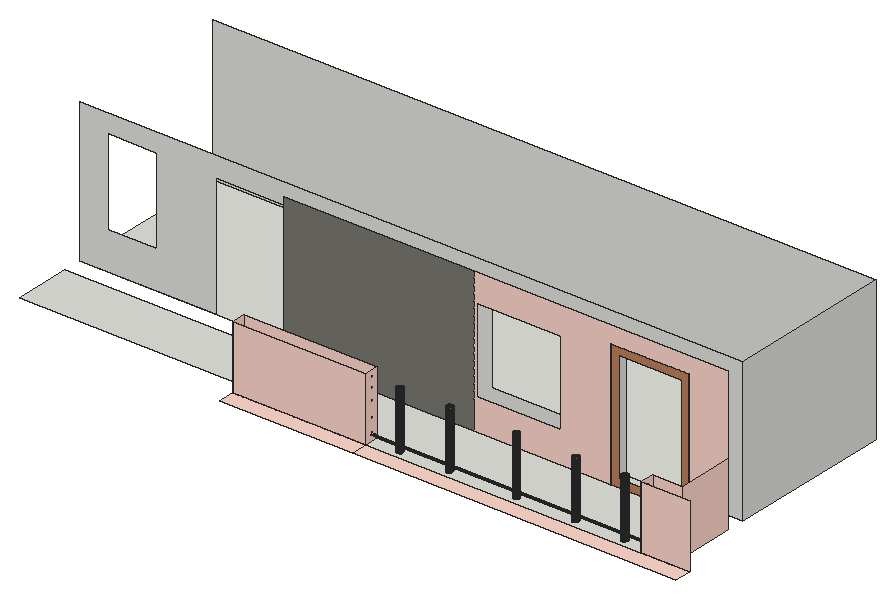
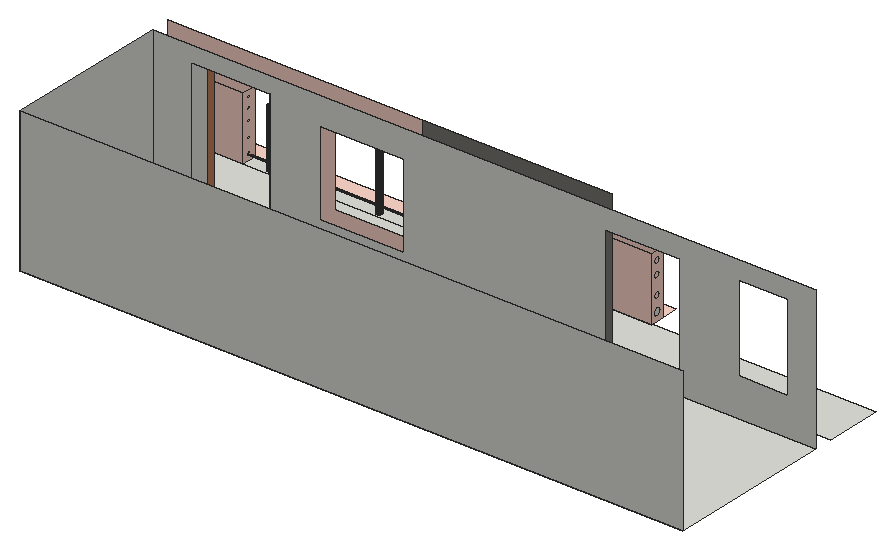
# SketchUp Ruby script. Lengths in inches.
U = 1.inch
M = Sketchup.active_model
def pt(a) = Geom::Point3d.new(a.map { |v| v * U })
def face(e, loops, mat)
  f = e.add_face(loops[0].map { |a| pt(a) })
  loops[1..].each { |l| e.add_face(l.map { |a| pt(a) }).erase! }
  f.material = f.back_material = mat if mat
  f
end
# faces: each face lists its corners as indices into pts; further lists are holes
def faces(e, pts, list, mat = nil) = list.each { |f| face(e, (f[0].is_a?(Array) ? f : [f]).map { |l| l.map { |i| pts[i] } }, mat) }
# xy, xz, yz: faces in a plane at the given z, y or x. An outline is a flat list of corners, or four numbers for a rectangle; further outlines are holes
def ring(l) = l.size == 4 ? [[l[0], l[1]], [l[2], l[1]], [l[2], l[3]], [l[0], l[3]]] : l.each_slice(2).to_a
def flat(e, list, mat, &to3) = list.each { |f| face(e, (f[0].is_a?(Array) ? f : [f]).map { |l| ring(l).map { |u, v| to3.(u, v) } }, mat) }
def xy(e, z, list, mat = nil) = flat(e, list, mat) { |x, y| [x, y, z] }
def xz(e, y, list, mat = nil) = flat(e, list, mat) { |x, z| [x, y, z] }
def yz(e, x, list, mat = nil) = flat(e, list, mat) { |y, z| [x, y, z] }
def lines(e, pts, list) = list.each { |a, b| e.add_line(pt(pts[a]), pt(pts[b])) }
# prism: a flat outline (further loops are holes) pulled along v
def prism(e, loops, v, mat = nil)
  f = face(e, loops, mat); d = Geom::Vector3d.new(v.map { |x| x * U })
  f.pushpull(f.normal.samedirection?(d) ? d.length : -d.length)
end
def box(e, o, s, mat = nil) = prism(e, [[o, [o[0] + s[0], o[1], o[2]], [o[0] + s[0], o[1] + s[1], o[2]], [o[0], o[1] + s[1], o[2]]]], [0, 0, s[2]], mat)
def at(x, y, z, deg = 0) = Geom::Transformation.translation(pt([x, y, z])) * Geom::Transformation.rotation(ORIGIN, Z_AXIS, deg.degrees)
def axes(o, x, y, z) = Geom::Transformation.new([*x, 0, *y, 0, *z, 0, *pt(o).to_a, 1])
def part(name) = M.definitions.add(name)
# library, detail: a bought-in or finely detailed component or shape, given as its bounding box
def library(name, o, s) = part(name).tap { |d| box(d.entities, o, s) }
def detail(e, o, s) = box(e.add_group.entities, o, s)
def put(e, d, t, mat = nil) = e.add_instance(d, t).tap { |i| i.material = mat if mat }
def group(e, t, mat = nil) = e.add_group.tap { |g| g.transformation = t; g.material = mat if mat }.entities
root = M.entities
M.materials.add("[Color B01]").color = [255, 216, 204]
M.materials.add("[Rough Square Concrete Block]").color = [123, 120, 113]
M.materials.add("[Wood Veneer 02]").color = [190, 128, 91]
xy(root,700.1875,[[1053.15,267.5625,1631.4,328.8],[[1631.4,267.5625,2829.41,328.8],[1753.2,288.65,1749.7,289.11,1746.45,290.45,1743.65,292.6,1741.51,295.4,1740.16,298.65,1739.7,302.15,1740.16,305.64,1741.51,308.9,1743.65,311.69,1746.45,313.84,1749.7,315.1875,1753.2,315.65,1756.69,315.1875,1759.95,313.84,1762.74,311.69,1764.89,308.9,1766.24,305.64,1766.7,302.15,1766.24,298.65,1764.89,295.4,1762.74,292.6,1759.95,290.45,1756.69,289.11],[2730.39,288.65,2726.89,289.11,2723.64,290.45,2720.84,292.6,2718.69,295.4,2717.35,298.65,2716.89,302.15,2717.35,305.64,2718.69,308.9,2720.84,311.69,2723.64,313.84,2726.89,315.1875,2730.39,315.65,2733.88,315.1875,2737.14,313.84,2739.93,311.69,2742.08,308.9,2743.43,305.64,2743.89,302.15,2743.43,298.65,2742.08,295.4,2739.93,292.6,2737.14,290.45,2733.88,289.11],[1968.45,288.65,1964.95,289.11,1961.7,290.45,1958.9,292.6,1956.76,295.4,1955.41,298.65,1954.95,302.15,1955.41,305.64,1956.76,308.9,1958.9,311.69,1961.7,313.84,1964.95,315.1875,1968.45,315.65,1971.94,315.1875,1975.2,313.84,1977.99,311.69,1980.14,308.9,1981.49,305.64,1981.95,302.15,1981.49,298.65,1980.14,295.4,1977.99,292.6,1975.2,290.45,1971.94,289.11],[2516.07,288.65,2512.58,289.11,2509.32,290.45,2506.53,292.6,2504.38,295.4,2503.03,298.65,2502.57,302.15,2503.03,305.64,2504.38,308.9,2506.53,311.69,2509.32,313.84,2512.58,315.1875,2516.07,315.65,2519.57,315.1875,2522.82,313.84,2525.62,311.69,2527.76,308.9,2529.11,305.64,2529.57,302.15,2529.11,298.65,2527.76,295.4,2525.62,292.6,2522.82,290.45,2519.57,289.11],[2258.76,288.65,2255.27,289.11,2252.01,290.45,2249.21,292.6,2247.07,295.4,2245.72,298.65,2245.26,302.15,2245.72,305.64,2247.07,308.9,2249.21,311.69,2252.01,313.84,2255.27,315.1875,2258.76,315.65,2262.25,315.1875,2265.51,313.84,2268.31,311.69,2270.45,308.9,2271.8,305.64,2272.26,302.15,2271.8,298.65,2270.45,295.4,2268.31,292.6,2265.51,290.45,2262.25,289.11]],[2829.41,267.5625,2962.22,328.8],[1753.2,288.65,1749.7,289.11,1746.45,290.45,1743.65,292.6,1741.51,295.4,1740.16,298.65,1739.7,302.15,1740.16,305.64,1741.51,308.9,1743.65,311.69,1746.45,313.84,1749.7,315.1875,1753.2,315.65,1756.69,315.1875,1759.95,313.84,1762.74,311.69,1764.89,308.9,1766.24,305.64,1766.7,302.15,1766.24,298.65,1764.89,295.4,1762.74,292.6,1759.95,290.45,1756.69,289.11],[1968.45,288.65,1964.95,289.11,1961.7,290.45,1958.9,292.6,1956.76,295.4,1955.41,298.65,1954.95,302.15,1955.41,305.64,1956.76,308.9,1958.9,311.69,1961.7,313.84,1964.95,315.1875,1968.45,315.65,1971.94,315.1875,1975.2,313.84,1977.99,311.69,1980.14,308.9,1981.49,305.64,1981.95,302.15,1981.49,298.65,1980.14,295.4,1977.99,292.6,1975.2,290.45,1971.94,289.11],
  [2258.76,288.65,2255.27,289.11,2252.01,290.45,2249.21,292.6,2247.07,295.4,2245.72,298.65,2245.26,302.15,2245.72,305.64,2247.07,308.9,2249.21,311.69,2252.01,313.84,2255.27,315.1875,2258.76,315.65,2262.25,315.1875,2265.51,313.84,2268.31,311.69,2270.45,308.9,2271.8,305.64,2272.26,302.15,2271.8,298.65,2270.45,295.4,2268.31,292.6,2265.51,290.45,2262.25,289.11],[2516.07,288.65,2512.58,289.11,2509.32,290.45,2506.53,292.6,2504.38,295.4,2503.03,298.65,2502.57,302.15,2503.03,305.64,2504.38,308.9,2506.53,311.69,2509.32,313.84,2512.58,315.1875,2516.07,315.65,2519.57,315.1875,2522.82,313.84,2525.62,311.69,2527.76,308.9,2529.11,305.64,2529.57,302.15,2529.11,298.65,2527.76,295.4,2525.62,292.6,2522.82,290.45,2519.57,289.11],[2730.39,288.65,2726.89,289.11,2723.64,290.45,2720.84,292.6,2718.69,295.4,2717.35,298.65,2716.89,302.15,2717.35,305.64,2718.69,308.9,2720.84,311.69,2723.64,313.84,2726.89,315.1875,2730.39,315.65,2733.88,315.1875,2737.14,313.84,2739.93,311.69,2742.08,308.9,2743.43,305.64,2743.89,302.15,2743.43,298.65,2742.08,295.4,2739.93,292.6,2737.14,290.45,2733.88,289.11],[77.93,328.8,2962.22,571.9],[2455.03,571.9,2794.72,653.97],
  [77.93,653.97,2962.22,1377.24]])
xy(root,700.1875,[[1053.15,195.0625,1631.4,267.5625],[1631.4,195.0625,3040.15,267.5625]],"[Color B01]")
xz(root,267.5625,[[1053.15,700.1875,1631.4,976.6875],[2829.41,700.1875,3040.15,976.6875]],"[Color B01]")
xz(root,328.8,[[1053.15,700.1875,1631.4,976.6875],[2829.41,700.1875,2962.22,976.6875]],"[Color B01]")
xz(root,571.9,[[[1857.32,700.1875,2455.03,700.1875,2455.03,1249.8125,2794.72,1249.8125,2794.72,700.1875,2962.22,700.1875,2962.22,1321.0625,1857.32,1321.0625],[1869.71,835.8,2235.65,1201.73]]],"[Color B01]")
xz(root,571.9,[[1031.89,700.1875,1857.32,1321.0625]],"[Rough Square Concrete Block]")
xz(root,571.9,[[[2455.03,700.1875,2794.72,1249.8125],[2488.22,733.38,2761.52,1216.62]]],"[Wood Veneer 02]")
xz(root,653.97,[[[77.93,700.1875,77.93,1321.0625,2962.22,1321.0625,2962.22,700.1875,2794.72,700.1875,2794.72,1249.8125,2455.03,1249.8125,2455.03,700.1875,998.42,700.1875,998.42,1230.86,670.44,1230.86,670.44,700.1875],[1869.71,835.8,2235.65,1201.73],[200.6,864.76,415.54,1240.57]]])
xz(root,1377.24,[[77.93,700.1875,2962.22,1321.0625]])
yz(root,1053.15,[[300.66,723.18,304.32,723.66,307.72,725.07,310.65,727.32,312.89,730.24,314.3,733.65,314.79,737.3,314.3,740.96,312.89,744.37,310.65,747.29,307.72,749.54,304.32,750.95,300.66,751.43,297,750.95,293.6,749.54,290.67,747.29,288.43,744.37,287.02,740.96,286.54,737.3,287.02,733.65,288.43,730.24,290.67,727.32,293.6,725.07,297,723.66]])
yz(root,1053.15,[[[267.5625,700.1875,328.8,976.6875],[300.66,924.24,304.32,924.72,307.72,926.13,310.65,928.38,312.89,931.3,314.3,934.71,314.79,938.37,314.3,942.02,312.89,945.43,310.65,948.35,307.72,950.6,304.32,952.01,300.66,952.49,297,952.01,293.6,950.6,290.67,948.35,288.43,945.43,287.02,942.02,286.54,938.37,287.02,934.71,288.43,931.3,290.67,928.38,293.6,926.13,297,924.72],[300.66,723.18,304.32,723.66,307.72,725.07,310.65,727.32,312.89,730.24,314.3,733.65,314.79,737.3,314.3,740.96,312.89,744.37,310.65,747.29,307.72,749.54,304.32,750.95,300.66,751.43,297,750.95,293.6,749.54,290.67,747.29,288.43,744.37,287.02,740.96,286.54,737.3,287.02,733.65,288.43,730.24,290.67,727.32,293.6,725.07,297,723.66],[300.66,867.43,304.32,867.91,307.72,869.32,310.65,871.57,312.89,874.49,314.3,877.9,314.79,881.55,314.3,885.21,312.89,888.62,310.65,891.54,307.72,893.79,304.32,895.2,300.66,895.68,297,895.2,293.6,893.79,290.67,891.54,288.43,888.62,287.02,885.21,286.54,881.55,287.02,877.9,288.43,874.49,290.67,871.57,293.6,869.32,297,867.91],[300.66,787.68,304.32,788.16,307.72,789.57,310.65,791.82,312.89,794.74,314.3,798.15,314.79,801.8,314.3,805.46,312.89,808.87,310.65,811.79,307.72,814.04,304.32,815.45,300.66,815.93,297,815.45,293.6,814.04,290.67,811.79,288.43,808.87,287.02,805.46,286.54,801.8,287.02,798.15,288.43,794.74,290.67,791.82,293.6,789.57,297,788.16]]],"[Color B01]")
yz(root,1631.4,[[[267.5625,700.1875,328.8,976.6875],[299.91,944.27,298.09,944.51,296.38,945.21,294.92,946.33,293.8,947.8,293.09,949.5,292.85,951.33,293.09,953.16,293.8,954.86,294.92,956.32,296.38,957.44,298.09,958.15,299.91,958.39,301.74,958.15,303.44,957.44,304.91,956.32,306.03,954.86,306.73,953.16,306.98,951.33,306.73,949.5,306.03,947.8,304.91,946.33,303.44,945.21,301.74,944.51],[299.91,899.83,298.09,900.07,296.38,900.77,294.92,901.9,293.8,903.36,293.09,905.0625,292.85,906.89,293.09,908.72,293.8,910.42,294.92,911.88,296.38,913.01,298.09,913.71,299.91,913.95,301.74,913.71,303.44,913.01,304.91,911.88,306.03,910.42,306.73,908.72,306.98,906.89,306.73,905.0625,306.03,903.36,304.91,901.9,303.44,900.77,301.74,900.07],[299.91,724.45,298.09,724.69,296.38,725.4,294.92,726.52,293.8,727.98,293.09,729.6875,292.85,731.52,293.09,733.34,293.8,735.05,294.92,736.51,296.38,737.63,298.09,738.34,299.91,738.58,301.74,738.34,303.44,737.63,304.91,736.51,306.03,735.05,306.73,733.34,306.98,731.52,306.73,729.6875,306.03,727.98,304.91,726.52,303.44,725.4,301.74,724.69],[299.91,851.52,298.09,851.76,296.38,852.46,294.92,853.58,293.8,855.05,293.09,856.75,292.85,858.58,293.09,860.41,293.8,862.11,294.92,863.57,296.38,864.69,298.09,865.4,299.91,865.64,301.74,865.4,303.44,864.69,304.91,863.57,306.03,862.11,306.73,860.41,306.98,858.58,306.73,856.75,306.03,855.05,304.91,853.58,303.44,852.46,301.74,851.76],[299.91,784.77,298.09,785.01,296.38,785.71,294.92,786.83,293.8,788.3,293.09,790,292.85,791.83,293.09,793.66,293.8,795.36,294.92,796.82,296.38,797.94,298.09,798.65,299.91,798.89,301.74,798.65,303.44,797.94,304.91,796.82,306.03,795.36,306.73,793.66,306.98,791.83,306.73,790,306.03,788.3,304.91,786.83,303.44,785.71,301.74,785.01]]],"[Color B01]")
yz(root,2455.03,[[571.9,700.1875,653.97,1249.8125]])
yz(root,2794.72,[[571.9,700.1875,653.97,1249.8125]])
yz(root,2829.41,[[299.91,724.45,301.74,724.69,303.44,725.4,304.91,726.52,306.03,727.98,306.73,729.6875,306.98,731.52,306.73,733.34,306.03,735.05,304.91,736.51,303.44,737.63,301.74,738.34,299.91,738.58,298.09,738.34,296.38,737.63,294.92,736.51,293.8,735.05,293.09,733.34,292.85,731.52,293.09,729.6875,293.8,727.98,294.92,726.52,296.38,725.4,298.09,724.69]])
yz(root,2829.41,[[[267.5625,700.1875,328.8,976.6875],[299.91,724.45,301.74,724.69,303.44,725.4,304.91,726.52,306.03,727.98,306.73,729.6875,306.98,731.52,306.73,733.34,306.03,735.05,304.91,736.51,303.44,737.63,301.74,738.34,299.91,738.58,298.09,738.34,296.38,737.63,294.92,736.51,293.8,735.05,293.09,733.34,292.85,731.52,293.09,729.6875,293.8,727.98,294.92,726.52,296.38,725.4,298.09,724.69],[299.91,899.83,301.74,900.07,303.44,900.77,304.91,901.9,306.03,903.36,306.73,905.0625,306.98,906.89,306.73,908.72,306.03,910.42,304.91,911.88,303.44,913.01,301.74,913.71,299.91,913.95,298.09,913.71,296.38,913.01,294.92,911.88,293.8,910.42,293.09,908.72,292.85,906.89,293.09,905.0625,293.8,903.36,294.92,901.9,296.38,900.77,298.09,900.07],[299.91,944.27,301.74,944.51,303.44,945.21,304.91,946.33,306.03,947.8,306.73,949.5,306.98,951.33,306.73,953.16,306.03,954.86,304.91,956.32,303.44,957.44,301.74,958.15,299.91,958.39,298.09,958.15,296.38,957.44,294.92,956.32,293.8,954.86,293.09,953.16,292.85,951.33,293.09,949.5,293.8,947.8,294.92,946.33,296.38,945.21,298.09,944.51],[299.91,851.52,301.74,851.76,303.44,852.46,304.91,853.58,306.03,855.05,306.73,856.75,306.98,858.58,306.73,860.41,306.03,862.11,304.91,863.57,303.44,864.69,301.74,865.4,299.91,865.64,298.09,865.4,296.38,864.69,294.92,863.57,293.8,862.11,293.09,860.41,292.85,858.58,293.09,856.75,293.8,855.05,294.92,853.58,296.38,852.46,298.09,851.76],[299.91,784.77,301.74,785.01,303.44,785.71,304.91,786.83,306.03,788.3,306.73,790,306.98,791.83,306.73,793.66,306.03,795.36,304.91,796.82,303.44,797.94,301.74,798.65,299.91,798.89,298.09,798.65,296.38,797.94,294.92,796.82,293.8,795.36,293.09,793.66,292.85,791.83,293.09,790,293.8,788.3,294.92,786.83,296.38,785.71,298.09,785.01]]],"[Color B01]")
yz(root,2962.22,[[653.97,700.1875,1377.24,1321.0625]])
yz(root,2962.22,[[328.8,700.1875,571.9,976.6875]],"[Color B01]")
p = [[1749.7,289.11,700.1875],[1753.2,288.65,700.1875],[1753.2,288.65,949.9375],[1749.7,289.11,949.9375],[1756.69,289.11,700.1875],[1756.69,289.11,949.9375],
  [1964.95,289.11,700.1875],[1968.45,288.65,700.1875],[1968.45,288.65,952.5625],[1964.95,289.11,952.5625],[1971.94,289.11,700.1875],[1971.94,289.11,952.5625],
  [2255.27,289.11,700.1875],[2258.76,288.65,700.1875],[2258.76,288.65,951.33],[2255.27,289.11,951.33],[2262.25,289.11,700.1875],[2262.25,289.11,951.33],
  [2512.58,289.11,700.1875],[2516.07,288.65,700.1875],[2516.07,288.65,949.5],[2512.58,289.11,949.5],[2519.57,289.11,700.1875],[2519.57,289.11,949.5],
  [2726.89,289.11,700.1875],[2730.39,288.65,700.1875],[2730.39,288.65,953.16],[2726.89,289.11,953.16],[2733.88,289.11,700.1875],[2733.88,289.11,953.16],
  [1746.45,290.45,700.1875],[1746.45,290.45,949.9375],[1759.95,290.45,700.1875],[1759.95,290.45,949.9375],[1961.7,290.45,700.1875],[1961.7,290.45,952.5625],
  [1975.2,290.45,700.1875],[1975.2,290.45,952.5625],[2252.01,290.45,700.1875],[2252.01,290.45,951.33],[2265.51,290.45,700.1875],[2265.51,290.45,951.33],
  [2509.32,290.45,700.1875],[2509.32,290.45,949.5],[2522.82,290.45,700.1875],[2522.82,290.45,949.5],[2723.64,290.45,700.1875],[2723.64,290.45,953.16],
  [2737.14,290.45,700.1875],[2737.14,290.45,953.16],[1743.65,292.6,700.1875],[1743.65,292.6,949.9375],[1762.74,292.6,700.1875],[1762.74,292.6,949.9375],
  [1958.9,292.6,700.1875],[1958.9,292.6,952.5625],[1977.99,292.6,700.1875],[1977.99,292.6,952.5625],[2249.21,292.6,700.1875],[2249.21,292.6,951.33],
  [2268.31,292.6,700.1875],[2268.31,292.6,951.33],[2506.53,292.6,700.1875],[2506.53,292.6,949.5],[2525.62,292.6,700.1875],[2525.62,292.6,949.5],
  [2720.84,292.6,700.1875],[2720.84,292.6,953.16],[2739.93,292.6,700.1875],[2739.93,292.6,953.16],[1741.51,295.4,700.1875],[1741.51,295.4,949.9375],
  [1764.89,295.4,700.1875],[1764.89,295.4,949.9375],[1956.76,295.4,700.1875],[1956.76,295.4,952.5625],[1980.14,295.4,700.1875],[1980.14,295.4,952.5625],
  [2247.07,295.4,700.1875],[2249.02,292.85,951.33],[2247.07,295.4,951.33],[2270.45,295.4,700.1875],[2270.45,295.4,951.33],[2268.5,292.85,951.33],
  [2504.38,295.4,700.1875],[2506.15,293.09,949.5],[2504.38,295.4,949.5],[2527.76,295.4,700.1875],[2527.76,295.4,949.5],[2526,293.09,949.5],
  [2718.69,295.4,700.1875],[2720.46,293.09,953.16],[2718.69,295.4,953.16],[2742.08,295.4,700.1875],[2742.08,295.4,953.16],[2740.31,293.09,953.16],
  [1740.16,298.65,700.1875],[1740.16,298.65,949.9375],[1766.24,298.65,700.1875],[1766.24,298.65,949.9375],[1955.41,298.65,700.1875],[1955.41,298.65,952.5625],
  [1981.49,298.65,700.1875],[1981.49,298.65,952.5625],[2245.72,298.65,700.1875],[2245.72,298.65,951.33],[2271.8,298.65,700.1875],[2271.8,298.65,951.33],
  [2503.03,298.65,700.1875],[2503.03,298.65,949.5],[2529.11,298.65,700.1875],[2529.11,298.65,949.5],[2717.35,298.65,700.1875],[2717.35,298.65,953.16],
  [2743.43,298.65,700.1875],[2743.43,298.65,953.16],[1739.7,302.15,700.1875],[1739.7,302.15,949.9375],[1766.7,302.15,700.1875],[1766.7,302.15,949.9375],
  [1954.95,302.15,700.1875],[1954.95,302.15,952.5625],[1981.95,302.15,700.1875],[1981.95,302.15,952.5625],[2245.26,302.15,700.1875],[2245.26,302.15,951.33],
  [2272.26,302.15,700.1875],[2272.26,302.15,951.33],[2502.57,302.15,700.1875],[2502.57,302.15,949.5],[2529.57,302.15,700.1875],[2529.57,302.15,949.5],
  [2716.89,302.15,700.1875],[2716.89,302.15,953.16],[2743.89,302.15,700.1875],[2743.89,302.15,953.16],[1740.16,305.64,700.1875],[1740.16,305.64,949.9375],
  [1766.24,305.64,700.1875],[1766.24,305.64,949.9375],[1955.41,305.64,700.1875],[1955.41,305.64,952.5625],[1981.49,305.64,700.1875],[1981.49,305.64,952.5625],
  [2245.72,305.64,700.1875],[2245.72,305.64,951.33],[2271.8,305.64,700.1875],[2271.8,305.64,951.33],[2503.03,305.64,700.1875],[2503.03,305.64,949.5],
  [2529.11,305.64,700.1875],[2529.11,305.64,949.5],[2717.35,305.64,700.1875],[2717.35,305.64,953.16],[2743.43,305.64,700.1875],[2743.43,305.64,953.16],
  [1741.51,308.9,700.1875],[1741.51,308.9,949.9375],[1764.89,308.9,700.1875],[1764.89,308.9,949.9375],[1956.76,308.9,700.1875],[1956.76,308.9,952.5625],
  [1980.14,308.9,700.1875],[1980.14,308.9,952.5625],[2247.07,308.9,700.1875],[2246.27,306.98,951.33],[2247.07,308.9,951.33],[2270.45,308.9,700.1875],
  [2270.45,308.9,951.33],[2271.25,306.98,951.33],[2504.38,308.9,700.1875],[2503.49,306.73,949.5],[2504.38,308.9,949.5],[2527.76,308.9,700.1875],
  [2527.76,308.9,949.5],[2528.66,306.73,949.5],[2718.69,308.9,700.1875],[2717.8,306.73,953.16],[2718.69,308.9,953.16],[2742.08,308.9,700.1875],
  [2742.08,308.9,953.16],[2742.97,306.73,953.16],[1743.65,311.69,700.1875],[1743.65,311.69,949.9375],[1762.74,311.69,700.1875],[1762.74,311.69,949.9375],
  [1958.9,311.69,700.1875],[1958.9,311.69,952.5625],[1977.99,311.69,700.1875],[1977.99,311.69,952.5625],[2249.21,311.69,700.1875],[2249.21,311.69,951.33],
  [2268.31,311.69,700.1875],[2268.31,311.69,951.33],[2506.53,311.69,700.1875],[2506.53,311.69,949.5],[2525.62,311.69,700.1875],[2525.62,311.69,949.5],
  [2720.84,311.69,700.1875],[2720.84,311.69,953.16],[2739.93,311.69,700.1875],[2739.93,311.69,953.16],[1746.45,313.84,700.1875],[1746.45,313.84,949.9375],
  [1759.95,313.84,700.1875],[1759.95,313.84,949.9375],[1961.7,313.84,700.1875],[1961.7,313.84,952.5625],[1975.2,313.84,700.1875],[1975.2,313.84,952.5625],
  [2252.01,313.84,700.1875],[2252.01,313.84,951.33],[2265.51,313.84,700.1875],[2265.51,313.84,951.33],[2509.32,313.84,700.1875],[2509.32,313.84,949.5],
  [2522.82,313.84,700.1875],[2522.82,313.84,949.5],[2723.64,313.84,700.1875],[2723.64,313.84,953.16],[2737.14,313.84,700.1875],[2737.14,313.84,953.16],
  [1749.7,315.1875,700.1875],[1749.7,315.1875,949.9375],[1756.69,315.1875,700.1875],[1756.69,315.1875,949.9375],[1964.95,315.1875,700.1875],[1964.95,315.1875,952.5625],
  [1971.94,315.1875,700.1875],[1971.94,315.1875,952.5625],[2255.27,315.1875,700.1875],[2255.27,315.1875,951.33],[2262.25,315.1875,700.1875],[2262.25,315.1875,951.33],
  [2512.58,315.1875,700.1875],[2512.58,315.1875,949.5],[2519.57,315.1875,700.1875],[2519.57,315.1875,949.5],[2726.89,315.1875,700.1875],[2726.89,315.1875,953.16],
  [2733.88,315.1875,700.1875],[2733.88,315.1875,953.16],[1753.2,315.65,700.1875],[1753.2,315.65,949.9375],[1968.45,315.65,700.1875],[1968.45,315.65,952.5625],
  [2258.76,315.65,700.1875],[2258.76,315.65,951.33],[2516.07,315.65,700.1875],[2516.07,315.65,949.5],[2730.39,315.65,700.1875],[2730.39,315.65,953.16],
  [2829.41,299.91,724.45],[2829.41,298.09,724.69],[1631.4,298.09,724.69],[1631.4,299.91,724.45],[2829.41,301.74,724.69],[1631.4,301.74,724.69],
  [2829.41,296.38,725.4],[1631.4,296.38,725.4],[2829.41,303.44,725.4],[1631.4,303.44,725.4],[2829.41,294.92,726.52],[1631.4,294.92,726.52],
  [2829.41,304.91,726.52],[1631.4,304.91,726.52]]
faces(root,p,[[0,1,2,3],[1,4,5,2],[6,7,8,9],[7,10,11,8],[12,13,14,15],[13,16,17,14],[18,19,20,21],[19,22,23,20],
  [24,25,26,27],[25,28,29,26],[30,0,3,31],[4,32,33,5],[34,6,9,35],[10,36,37,11],[38,12,15,39],[16,40,41,17],
  [42,18,21,43],[22,44,45,23],[46,24,27,47],[28,48,49,29],[50,30,31,51],[32,52,53,33],[54,34,35,55],[36,56,57,37],
  [58,38,39,59],[40,60,61,41],[62,42,43,63],[44,64,65,45],[66,46,47,67],[48,68,69,49],[70,50,51,71],[52,72,73,53],
  [74,54,55,75],[56,76,77,57],[78,58,59,79,80],[60,81,82,83,61],[84,62,63,85,86],[64,87,88,89,65],[90,66,67,91,92],[68,93,94,95,69],
  [96,70,71,97],[72,98,99,73],[100,74,75,101],[76,102,103,77],[104,78,80,105],[81,106,107,82],[108,84,86,109],[87,110,111,88],
  [112,90,92,113],[93,114,115,94],[116,96,97,117],[98,118,119,99],[120,100,101,121],[102,122,123,103],[124,104,105,125],[106,126,127,107],
  [128,108,109,129],[110,130,131,111],[132,112,113,133],[114,134,135,115],[136,116,117,137],[118,138,139,119],[140,120,121,141],[122,142,143,123],
  [144,124,125,145],[126,146,147,127],[148,128,129,149],[130,150,151,131],[152,132,133,153],[134,154,155,135],[156,136,137,157],[138,158,159,139],
  [160,140,141,161],[142,162,163,143],[164,144,145,165,166],[146,167,168,169,147],[170,148,149,171,172],[150,173,174,175,151],[176,152,153,177,178],[154,179,180,181,155],
  [182,156,157,183],[158,184,185,159],[186,160,161,187],[162,188,189,163],[190,164,166,191],[167,192,193,168],[194,170,172,195],[173,196,197,174],
  [198,176,178,199],[179,200,201,180],[202,182,183,203],[184,204,205,185],[206,186,187,207],[188,208,209,189],[210,190,191,211],[192,212,213,193],
  [214,194,195,215],[196,216,217,197],[218,198,199,219],[200,220,221,201],[222,202,203,223],[204,224,225,205],[226,206,207,227],[208,228,229,209],
  [230,210,211,231],[212,232,233,213],[234,214,215,235],[216,236,237,217],[238,218,219,239],[220,240,241,221],[242,222,223,243],[224,242,243,225],
  [244,226,227,245],[228,244,245,229],[246,230,231,247],[232,246,247,233],[248,234,235,249],[236,248,249,237],[250,238,239,251],[240,250,251,241],
  [252,253,254,255],[256,252,255,257],[253,258,259,254],[260,256,257,261],[258,262,263,259],[264,260,261,265]],"[Wood Veneer 02]")
